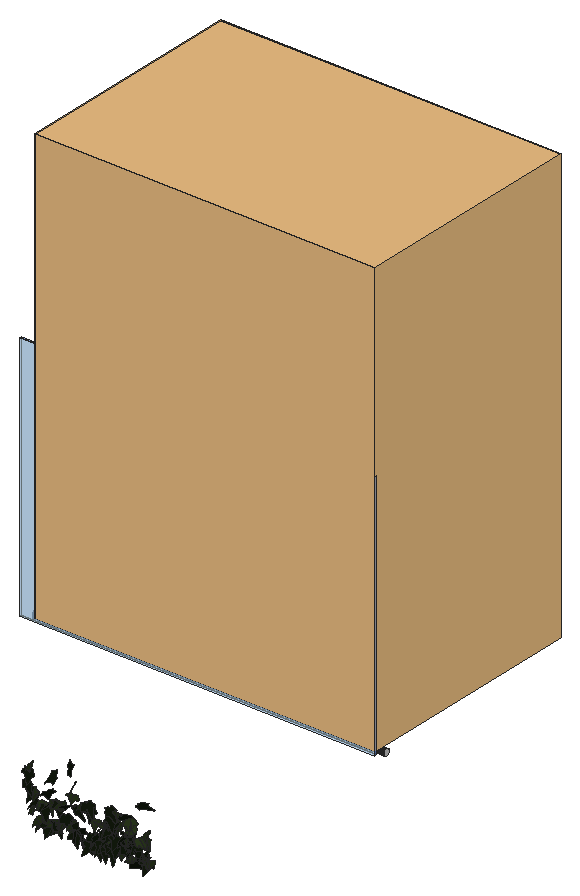
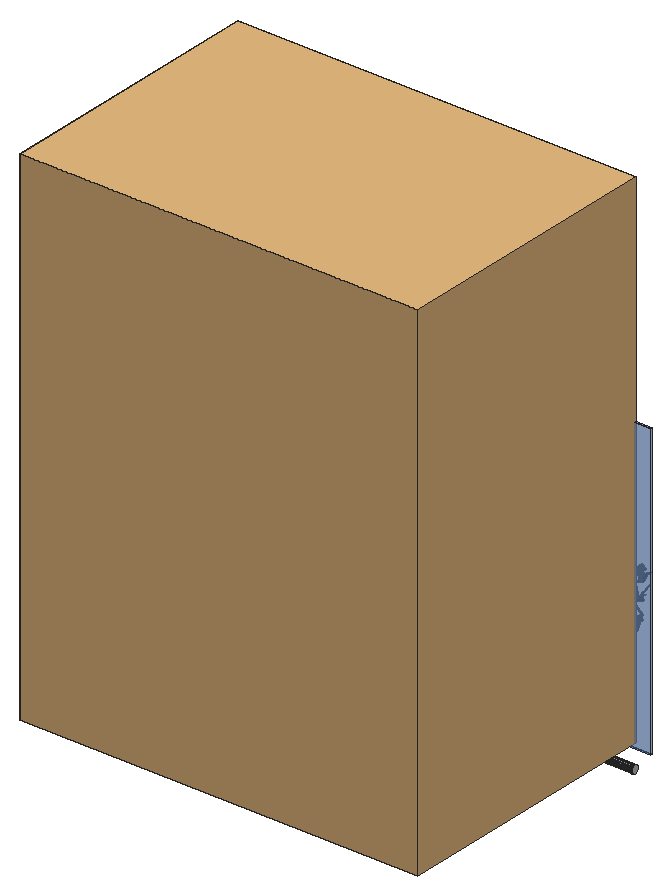
# SketchUp Ruby script. Lengths in inches.
U = 1.inch
M = Sketchup.active_model
def pt(a) = Geom::Point3d.new(a.map { |v| v * U })
def face(e, loops, mat)
  f = e.add_face(loops[0].map { |a| pt(a) })
  loops[1..].each { |l| e.add_face(l.map { |a| pt(a) }).erase! }
  f.material = f.back_material = mat if mat
  f
end
# faces: each face lists its corners as indices into pts; further lists are holes
def faces(e, pts, list, mat = nil) = list.each { |f| face(e, (f[0].is_a?(Array) ? f : [f]).map { |l| l.map { |i| pts[i] } }, mat) }
# xy, xz, yz: faces in a plane at the given z, y or x. An outline is a flat list of corners, or four numbers for a rectangle; further outlines are holes
def ring(l) = l.size == 4 ? [[l[0], l[1]], [l[2], l[1]], [l[2], l[3]], [l[0], l[3]]] : l.each_slice(2).to_a
def flat(e, list, mat, &to3) = list.each { |f| face(e, (f[0].is_a?(Array) ? f : [f]).map { |l| ring(l).map { |u, v| to3.(u, v) } }, mat) }
def xy(e, z, list, mat = nil) = flat(e, list, mat) { |x, y| [x, y, z] }
def xz(e, y, list, mat = nil) = flat(e, list, mat) { |x, z| [x, y, z] }
def yz(e, x, list, mat = nil) = flat(e, list, mat) { |y, z| [x, y, z] }
def lines(e, pts, list) = list.each { |a, b| e.add_line(pt(pts[a]), pt(pts[b])) }
# prism: a flat outline (further loops are holes) pulled along v
def prism(e, loops, v, mat = nil)
  f = face(e, loops, mat); d = Geom::Vector3d.new(v.map { |x| x * U })
  f.pushpull(f.normal.samedirection?(d) ? d.length : -d.length)
end
def box(e, o, s, mat = nil) = prism(e, [[o, [o[0] + s[0], o[1], o[2]], [o[0] + s[0], o[1] + s[1], o[2]], [o[0], o[1] + s[1], o[2]]]], [0, 0, s[2]], mat)
def at(x, y, z, deg = 0) = Geom::Transformation.translation(pt([x, y, z])) * Geom::Transformation.rotation(ORIGIN, Z_AXIS, deg.degrees)
def axes(o, x, y, z) = Geom::Transformation.new([*x, 0, *y, 0, *z, 0, *pt(o).to_a, 1])
def part(name) = M.definitions.add(name)
# library, detail: a bought-in or finely detailed component or shape, given as its bounding box
def library(name, o, s) = part(name).tap { |d| box(d.entities, o, s) }
def detail(e, o, s) = box(e.add_group.entities, o, s)
def put(e, d, t, mat = nil) = e.add_instance(d, t).tap { |i| i.material = mat if mat }
def group(e, t, mat = nil) = e.add_group.tap { |g| g.transformation = t; g.material = mat if mat }.entities
root = M.entities
M.materials.add("Glass Rail Metal").color = [192, 192, 192]
M.materials.add("[Translucent Glass Blue]").color = [100, 149, 237]
M.materials["[Translucent Glass Blue]"].alpha = 0.5
M.materials.add("[Translucent Glass Safety]").color = [204, 235, 244]
M.materials["[Translucent Glass Safety]"].alpha = 0.5
M.materials.add("efeu1").color = [18, 25, 13]
M.materials.add("efeu2").color = [43, 57, 29]
c1 = part("ivyleaf_9")
p = [[1.54,2.16,1.25],[1.36,2.04,1.19],[-0.21,0.99,0.68],[-0.71,1.11,0.82],[-0.85,0.86,0.67],[-0.8,0.17,0.21],
  [-0.9,-0.01,0.1],[-0.67,-0.16,-0.02],[-0.08,-0.08,-0.05],[-0.03,-0.6,-0.4],[0.65,-0.88,-0.66],[0.83,-0.6,-0.49],
  [1.29,-0.42,-0.43],[1.8125,-0.07,-0.26],[1.21,0.44,0.15]]
faces(c1.entities,p,[[0,1,2,3,4,5,6,7,8,9,10,11,12,13,14]],"efeu1")
c2 = part("ivyleaf_10")
p = [[0,0.5,-0.03],[-0.0625,2.02,-0.43],[-0.19,2.01,-0.46],[-0.54,1.05,-0.29],[-0.52,0.625,-0.18],[-0.83,0.76,-0.28],
  [-1.16,0.64,-0.33],[-1.15,0.33,-0.24],[-0.77,-0.39,0.02],[-0.3,-0.51,0.16],[0.04,-0.48,0.23],[-0.02,2.01,-0.4375],
  [-0.06,2.01,-0.43],[0.04,-0.49,0.23],[0.67,-0.49,0.14],[1.38,0.36,-0.2],[1.375,0.51,-0.24],[0.81,0.65,-0.19],
  [0.62,0.59,-0.15],[0.6,1.09,-0.28],[0.5,1.23,-0.31]]
faces(c2.entities,p,[[0,1,2,3,4,5,6,7,8,9,10],[11,12,0,13,14,15,16,17,18,19,20]],"efeu2")
c3 = library("Palm+in+pot",[-44.1,-44.03,0.04],[106.77,95.72,88.04])
prism(root,[[[506.55,181.67,254.4375],[506.55,181.84,254.35],[506.55,181.98,254.2],[506.55,182.09,254.02],[506.55,182.16,253.8125],[506.55,182.17,253.59],[506.55,182.14,253.375],[506.55,182.0625,253.18],[506.55,181.94,253.01],[506.55,181.79,252.88],[506.55,181.61,252.8],[506.55,181.43,252.78],[506.55,181.25,252.82],[506.55,181.08,252.91],[506.55,180.93,253.06],[506.55,180.83,253.24],[506.55,180.76,253.45],[506.55,180.75,253.67],[506.55,180.78,253.88],[506.55,180.86,254.09],[506.55,180.98,254.26],[506.55,181.13,254.38],[506.55,181.3,254.46],[506.55,181.49,254.48]]],[89.11,0,0],"Glass Rail Metal")
xy(root,254.7,[[506.22,177.2,595.99,177.79]],"[Translucent Glass Blue]")
xy(root,318.08,[[506.22,177.2,595.99,177.79]],"[Translucent Glass Blue]")
xz(root,177.2,[[506.22,254.7,595.99,318.08]],"[Translucent Glass Safety]")
xz(root,177.79,[[506.22,254.7,595.99,318.08]],"[Translucent Glass Blue]")
yz(root,506.22,[[177.2,254.7,177.79,318.08]],"[Translucent Glass Blue]")
yz(root,595.99,[[177.2,254.7,177.79,318.08]],"[Translucent Glass Blue]")
put(root,c1,axes([550.24,130.16,247.6875],[0.09934,-1.04431,-0.03336],[-0.02326,0.03129,-1.04883],[1.04459,0.10002,-0.02018]))
put(root,c1,axes([552.99,129.83,255.84],[-0.98011,0.38799,0.10195],[-0.09768,0.03022,-1.05409],[-0.38909,-0.98494,0.00782]))
put(root,c2,axes([571.6,130.2,247.97],[0.10661,-0.93081,0.4596],[0.10935,-0.44938,-0.93547],[1.03232,0.14373,0.05162]))
put(root,c2,axes([568.95,129.58,252.98],[-1.03024,0.12903,0.14532],[-0.14137,0.04033,-1.03805],[-0.13335,-1.03965,-0.02224]))
put(root,c1,axes([567.14,130.2,249.14],[-1.00045,-0.31834,0.02077],[-0.01948,-0.00727,-1.04987],[0.31842,-1.00064,0.00102]))
put(root,c1,axes([566.3,130.3,247.05],[-0.94363,-0.22886,-0.35753],[0.40475,-0.22235,-0.92594],[0.12797,-0.98429,0.2923]))
put(root,c1,axes([564.81,130.36,244.37],[-0.8856,-0.51614,-0.03288],[0.13113,-0.16102,-1.00431],[0.50028,-0.87146,0.20504]))
put(root,c2,axes([557.65,129.82,253.03],[-0.9508,-0.35541,0.30029],[-0.26159,-0.15666,-1.01368],[0.38479,-0.98471,0.05289]))
put(root,c2,axes([555.12,129.88,246.03],[0.2577,-1.02396,-0.05486],[-0.00277,0.05587,-1.05584],[1.02543,0.25749,0.01093]))
put(root,c2,axes([570.09,129.83,251.39],[0.15346,-1.03516,-0.1201],[-0.03109,0.11679,-1.04638],[1.04164,0.15599,-0.01354]))
put(root,c2,axes([548.8,129.43,244.65],[-0.29578,-0.77346,-0.63277],[0.29896,0.56119,-0.82572],[0.95355,-0.41587,0.06261]))
put(root,c1,axes([561.11,129.98,252.27],[0.06997,-0.99633,-0.43816],[0.1214,0.44347,-0.98902],[1.08163,0.01468,0.13935]))
put(root,c1,axes([566.86,130.26,251.14],[0.0567,-1.02927,-0.01108],[0.02641,0.01255,-1.03047],[1.02899,0.05639,0.02705]))
put(root,c1,axes([569.26,130.05,251.66],[-0.88669,0.40318,-0.38442],[0.32838,-0.20543,-0.97289],[-0.45,-0.94435,0.04751]))
put(root,c2,axes([569.13,129.95,250.08],[0.50057,-0.93252,-0.02492],[0.03234,0.04561,-1.05719],[0.93229,0.49911,0.05005]))
put(root,c1,axes([545.99,130.43,254.45],[-0.09848,-1.02006,0.18085],[-0.02567,-0.17921,-1.02477],[1.03565,-0.10144,-0.0082]))
put(root,c1,axes([568.11,130.33,245.47],[-0.19213,-1.02505,-0.02846],[-0.00573,0.03003,-1.04284],[1.02543,-0.19189,-0.01117]))
put(root,c1,axes([557.15,129.06,259.48],[0.1044,0.34296,-1.03239],[-0.9038,0.60458,0.10944],[0.60547,0.84333,0.34139]))
put(root,c1,axes([571.29,129.55,246.63],[0.29839,-0.08644,1.07907],[1.08247,0.01167,-0.29839],[0.01175,1.11951,0.08643]))
put(root,c1,axes([570.63,129.35,253.07],[0.79554,0.6998,-0.06753],[-0.03683,-0.06035,-1.05932],[-0.70209,0.79612,-0.02094]))
put(root,c1,axes([561.56,130.56,243.1875],[-0.70211,-0.7243,0.2139],[-0.05539,-0.24189,-1.00087],[0.7532,-0.69296,0.12579]))
put(root,c2,axes([571.95,129.85,252.26],[0.83512,0.66517,-0.01359],[-0.06187,0.05593,-1.06448],[-0.66242,0.83336,0.08228]))
put(root,c1,axes([563.97,130.14,243.72],[-0.30671,-0.89186,-0.40394],[0.14247,0.37813,-0.94307],[0.96865,-0.33801,0.0108]))
put(root,c1,axes([545.68,130.13,251.9375],[0.37961,-0.97219,-0.12719],[-0.028,0.12558,-1.04349],[0.98007,0.38015,0.01945]))
put(root,c2,axes([551.5625,130.22,248.26],[-0.56597,0.43778,-0.75759],[0.45618,-0.62229,-0.7004],[-0.74665,-0.71205,0.14633]))
put(root,c1,axes([568.4,130.51,246.99],[-0.65794,-0.79879,0.01773],[0.06576,-0.07703,-1.03005],[0.79627,-0.65366,0.09972]))
put(root,c1,axes([548.24,130.03,248.86],[-0.89328,0.47822,-0.14667],[0.1075,-0.10964,-1.01222],[-0.48852,-0.89858,0.04545]))
put(root,c1,axes([566.43,130.52,245.88],[-0.38609,-0.95523,0.09098],[-0.00099,-0.09768,-1.02969],[0.95955,-0.38445,0.03555]))
put(root,c1,axes([566.67,129.27,249.59],[-0.14747,0.85178,0.56979],[-0.19449,0.54193,-0.86048],[-1.00616,-0.2296,0.08282]))
put(root,c1,axes([555.58,130.11,247.46],[0.04784,-0.93068,-0.40341],[0.02332,0.40476,-0.93103],[1.01408,0.0346,0.04044]))
put(root,c1,axes([561.63,130.41,251.24],[-0.22718,-1.00478,-0.11456],[0.00067,0.11726,-1.02984],[1.01129,-0.2258,-0.02505]))
put(root,c2,axes([548.16,129.26,250.43],[0.08731,-0.3789,-0.99376],[0.00491,0.99724,-0.37979],[1.06354,0.0265,0.08333]))
put(root,c1,axes([565.15,130.1,247.03],[0.43038,-0.89576,-0.24795],[-0.05593,0.24779,-0.99226],[0.92776,0.43047,0.05521]))
put(root,c2,axes([576.23,129.625,244.88],[0.56664,-0.10726,-0.85706],[-0.65733,0.6114,-0.51111],[0.56033,0.82572,0.26711]))
put(root,c2,axes([565.6,129.78,244.29],[0.72786,-0.56503,-0.47277],[-0.2147,0.47305,-0.89592],[0.70475,0.72767,0.21533]))
put(root,c2,axes([572.62,130.12,243.38],[-0.32749,-0.02674,0.99814],[-0.95098,-0.31185,-0.32037],[0.30437,-1.00314,0.07299]))
put(root,c1,axes([566.69,130.13,253.07],[0.31485,-0.95105,-0.3112],[0.03288,0.3359,-0.99326],[1.00013,0.28835,0.13063]))
put(root,c1,axes([546.93,130.73,250.14],[-0.42065,-0.86898,0.32729],[-0.07642,-0.32569,-0.96296],[0.92542,-0.42189,0.06925]))
put(root,c2,axes([557.26,129.83,246.52],[-0.09862,-0.99063,-0.37102],[0.12773,0.35875,-0.99183],[1.05009,-0.13668,0.08579]))
put(root,c2,axes([572.19,130.26,249.91],[0.50779,0.551,0.72978],[-0.50399,-0.52789,0.74925],[0.76301,-0.71538,0.00922]))
put(root,c1,axes([550.91,130.58,243.86],[-0.43171,-0.93763,-0.01567],[0.0485,-0.0051,-1.03121],[0.9365,-0.43197,0.04618]))
put(root,c2,axes([560.18,129.84,251.85],[-0.4836,-0.88252,-0.33517],[0.13583,0.30762,-1.00597],[0.9342,-0.50157,-0.02724]))
put(root,c2,axes([554.5,130.04,249.96],[-0.30229,-1.00367,-0.10117],[0.0285,0.09708,-1.04821],[1.00836,-0.30363,-0.00071]))
put(root,c1,axes([572.55,129.93,248.24],[-0.72246,0.73124,0.0075],[-0.00606,0.00456,-1.02794],[-0.73125,-0.72248,0.0011]))
put(root,c2,axes([574.5,129.75,248.84],[0.67457,0.59612,0.56255],[0.36186,0.43713,-0.89713],[-0.73545,0.76185,0.07457]))
put(root,c1,axes([551.11,129.6875,251.72],[0.3859,0.93418,-0.24925],[-0.10291,-0.22716,-1.01071],[-0.96136,0.3993,0.00814]))
put(root,c1,axes([553.16,130.21,244.79],[0.43009,-0.90853,-0.30046],[-0.13504,0.26849,-1.00517],[0.94735,0.45074,-0.00687]))
put(root,c1,axes([565.18,130.51,243.32],[-0.09038,-0.99865,-0.13127],[0.0749,0.12477,-1.00076],[1.00445,-0.09916,0.06281]))
put(root,c1,axes([573.55,130.59,247.3125],[-0.90884,-0.46811,-0.04788],[0.04546,0.01629,-1.02229],[0.46835,-0.90996,0.00632]))
put(root,c1,axes([573.58,130.05,245.82],[0.73663,-0.69796,-0.23578],[-0.06524,0.27031,-1.00401],[0.73382,0.72467,0.14742]))
put(root,c1,axes([564.57,129.51,247.99],[-0.07502,0.97908,0.3179],[-0.14942,0.30501,-0.97464],[-1.01849,-0.11686,0.11957]))
put(root,c2,axes([549.67,130.31,248.26],[0.71288,0.31821,-0.67189],[-0.66784,-0.13488,-0.77246],[-0.32663,0.97028,0.11297]))
put(root,c1,axes([557.6,130.42,244.22],[-0.01445,-0.98694,-0.28146],[0.08974,0.27919,-0.9836],[1.02236,-0.03845,0.08236]))
put(root,c2,axes([572.05,129.8,251.24],[0.39448,-0.78842,-0.58895],[-0.05803,0.61477,-0.86184],[0.98239,0.3529,0.18558]))
put(root,c1,axes([565.52,130.83,248.27],[-0.12512,-0.40963,0.92801],[0.34423,-0.89671,-0.3494],[0.9542,0.26977,0.24773]))
put(root,c1,axes([553.6,130.53,249.55],[-0.16886,-0.98327,-0.21084],[0.05873,0.20378,-0.9974],[1.00391,-0.17732,0.02289]))
put(root,c1,axes([561.5,130.07,250.78],[0.705,-0.71626,-0.42276],[-0.28815,0.30954,-1.00496],[0.78021,0.76153,0.01086]))
put(root,c1,axes([576.14,130.05,246.39],[-0.73215,0.73903,0.00971],[-0.00851,0.00523,-1.04029],[-0.73904,-0.7322,0.00237]))
put(root,c2,axes([553.25,130.34,245.14],[0.72581,-0.56514,0.47445],[0.57285,0.01206,-0.86196],[0.46511,0.86704,0.32124]))
put(root,c1,axes([573.36,129.52,243.26],[0.62148,0.92076,0.13104],[0.07303,0.10881,-1.11087],[-0.92716,0.62576,0.00034]))
put(root,c1,axes([558.13,129.57,244.32],[0.13552,0.03149,-1.0264],[-0.8725,0.54947,-0.09834],[0.5415,0.87746,0.09842]))
put(root,c2,axes([564.92,130.07,247.33],[0.4751,-0.85711,-0.33513],[-0.0044,0.37503,-0.9654],[0.92029,0.44427,0.16839]))
put(root,c2,axes([552.51,130.125,249.82],[-0.93419,-0.01619,-0.47853],[0.47841,0.01137,-0.93433],[0.01959,-1.04956,-0.00274]))
put(root,c2,axes([549.15,130.1875,247.85],[-0.97172,-0.29226,0.14895],[-0.1504,-0.01691,-1.01436],[0.29152,-0.98292,-0.02683]))
put(root,c2,axes([575.86,130.41,250.68],[-0.00324,-1.03693,0.03783],[-0.01405,-0.03778,-1.03684],[1.03752,-0.00375,-0.01392]))
put(root,c1,axes([566.8125,130.77,243.17],[0.11776,-1.0127,0.1095],[0.00095,-0.11012,-1.01945],[1.0186,0.11718,-0.01171]))
put(root,c1,axes([557.48,129.43,254.48],[-0.01253,0.65977,0.8441],[0.02028,0.84416,-0.65951],[-1.07116,0.00827,-0.02236]))
put(root,c1,axes([571.49,130.27,248.78],[0.72539,-0.74514,-0.11981],[0.09076,0.2511,-1.01217],[0.74923,0.69101,0.23861]))
put(root,c2,axes([562.95,130.62,248.72],[-0.54099,-0.81162,0.33309],[-0.01016,-0.38551,-0.95584],[0.87725,-0.50498,0.19434]))
put(root,c1,axes([574.63,129.67,256.87],[0.99918,0.40498,0.44983],[0.40536,0.19702,-1.07777],[-0.44949,1.07792,0.02798]))
put(root,c1,axes([552.08,130.4,244.81],[0.77952,-0.63543,0.21329],[0.22294,-0.06272,-1.00164],[0.63211,0.80574,0.09024]))
put(root,c1,axes([561.97,130.47,245.39],[0.07395,-0.93447,-0.38706],[0.08161,0.39234,-0.93162],[1.00816,0.03678,0.1038]))
put(root,c2,axes([546.41,130.3,256.1],[0.04439,-1.03146,-0.17572],[-0.03298,0.17441,-1.03211],[1.0458,0.04928,-0.02509]))
put(root,c2,axes([576.04,130.46,244.95],[0.46544,-0.92877,-0.04513],[-0.00403,0.04845,-1.03871],[0.92985,0.4651,0.01808]))
put(root,c2,axes([576.38,130.04,248.875],[-0.38627,0.93003,0.29023],[-0.25128,0.20654,-0.99629],[-0.9413,-0.43678,0.14686]))
put(root,c1,axes([563.375,130.67,245.52],[-0.1422,0.58015,-0.82585],[0.09855,-0.82204,-0.59445],[-1.00444,-0.16279,0.05859]))
put(root,c2,axes([554.03,130.08,244.5],[0.4468,-0.8008,-0.51243],[-0.0153,0.56007,-0.88859],[0.9506,0.38541,0.22655]))
put(root,c1,axes([569.43,130.45,248.46],[0.7165,-0.46528,0.58847],[0.57612,-0.17992,-0.84372],[0.48049,0.90956,0.13413]))
put(root,c2,axes([553.21,130.45,244.72],[-0.16551,-0.98816,-0.04855],[0.01138,0.04732,-1.00192],[0.98929,-0.16586,0.0034]))
put(root,c1,axes([560.07,130.55,243.03],[0.57214,-0.80984,0.02263],[0.17429,0.09599,-0.97165],[0.79119,0.56448,0.19769]))
put(root,c1,axes([570.04,130.52,245.34],[0.42285,-0.89334,-0.27629],[-0.03644,0.28725,-0.98456],[0.93438,0.41548,0.08663]))
put(root,c2,axes([576.54,130.6,244.15],[-0.4656,-0.87306,0.18737],[-0.07952,-0.16994,-0.98941],[0.8894,-0.47225,0.00963]))
put(root,c1,axes([561.82,130.85,244.6],[0.15714,-1.01272,0.00254],[0.00023,-0.00253,-1.02483],[1.01272,0.15714,-0.00016]))
put(root,c1,axes([575.77,130.98,243.84],[-0.65474,-0.77245,-0.08162],[0.12008,0.00481,-1.00875],[0.76741,-0.65979,0.0882]))
put(root,c1,axes([550.98,129.98,248.65],[-0.13713,1.01208,0.06521],[-0.06236,0.05726,-1.0199],[-1.01226,-0.14063,0.054]))
put(root,c2,axes([557.03,130.27,244.4],[-0.127,-0.95611,-0.36612],[0.1127,0.35363,-0.96258],[1.01759,-0.15849,0.06092]))
put(root,c1,axes([557.2,130.54,246.49],[0.66035,-0.80385,-0.22151],[-0.13104,0.179,-1.04024],[0.82345,0.67312,0.0121]))
put(root,c2,axes([548.28,130.19,243.23],[0.35646,-0.77203,-0.55109],[-0.07338,0.56451,-0.83829],[0.9457,0.3348,0.14268]))
put(root,c2,axes([565.59,130.8125,248.38],[-0.17166,-0.00508,-1.008],[-0.97549,-0.25681,0.16741],[-0.254,0.98973,0.03827]))
put(root,c1,axes([557.83,130.53,249.82],[0.67655,-0.76888,-0.15854],[0.0511,0.25198,-1.00395],[0.78339,0.64758,0.20241]))
put(root,c1,axes([567.3,130.1875,248.89],[0.67735,-0.36285,-0.81506],[-0.73628,0.3506,-0.76795],[0.50386,1.0001,-0.02649]))
put(root,c1,axes([565.95,130.75,247.82],[0.10709,-0.17692,1.00541],[0.83153,-0.57133,-0.18911],[0.5922,0.83421,0.08371]))
put(root,c2,axes([546.85,130.53,246.27],[0.1122,-0.99591,-0.24169],[0.02968,0.24619,-1.00067],[1.02438,0.10195,0.05546]))
put(root,c2,axes([565.3,130.69,245.28],[0.1124,-1.02114,-0.04419],[-0.02913,0.04123,-1.02701],[1.02168,0.11352,-0.02442]))
put(root,c2,axes([572.04,130.54,247.77],[0.06373,-0.98569,-0.28303],[0.03234,0.28537,-0.98654],[1.02501,0.05228,0.04873]))
put(root,c2,axes([570.94,130.64,245.06],[0.8748,-0.54541,0.04342],[0.17788,0.20609,-0.99525],[0.51741,0.85129,0.26876]))
put(root,c1,axes([553.01,131.14,243.77],[-0.94144,-0.31371,0.20184],[-0.17823,-0.10309,-0.9915],[0.3277,-0.9573,0.04062]))
put(root,c2,axes([568.84,130.49,243.88],[-0.96023,0.28164,0.17703],[-0.16123,0.07902,-1.00023],[-0.29098,-0.97321,-0.02998]))
put(root,c2,axes([551.28,130.73,244.55],[-0.72499,-0.71478,0.07784],[-0.05228,-0.05784,-1.01809],[0.7171,-0.72686,0.00447]))
put(root,c1,axes([572.16,130.14,246.18],[-0.15318,0.9663,0.3158],[-0.22715,0.27876,-0.96313],[-0.99089,-0.21328,0.17197]))
put(root,c2,axes([551.84,130.92,243.89],[0.60508,-0.80814,0.14738],[0.12723,-0.08864,-1.00841],[0.81155,0.61643,0.04821]))
put(root,c2,axes([567.0625,130.56,246],[0.75491,0.68437,0.19408],[0.07366,0.20627,-1.01388],[-0.70754,0.75167,0.10152]))
put(root,c2,axes([565.04,130.5,245.34],[0.97215,-0.03657,-0.36736],[-0.31815,0.44192,-0.88592],[0.18728,0.9406,0.40195]))
put(root,c2,axes([551.34,131.02,243.55],[-0.36505,-0.92195,0.21443],[0.0047,-0.23158,-0.98771],[0.94654,-0.35441,0.0876]))
put(root,c1,axes([574.42,130.23,244.55],[0.78714,0.65891,0.10361],[0.08923,0.0548,-1.02642],[-0.66101,0.79204,-0.01518]))
put(root,c2,axes([560.95,130.7,243.62],[0.8726,-0.52387,-0.15282],[0.06629,0.38784,-0.951],[0.54166,0.79647,0.36257]))
put(root,c2,axes([550.81,130.95,242.86],[-0.15781,-1.0057,0.01739],[-0.01837,-0.01472,-1.01789],[1.00569,-0.15808,-0.01587]))
put(root,c2,axes([554.41,130.54,245.28],[0.07841,-0.87053,-0.59265],[-0.05489,0.59011,-0.87405],[1.05168,0.0957,-0.00143]))
put(root,c1,axes([565.84,130.7,247.38],[0.89522,-0.4395,-0.21401],[-0.1196,0.23604,-0.98507],[0.47398,0.88967,0.15563]))
put(root,c1,axes([559.61,130.25,243.2],[0.24724,0.24996,-0.93266],[-0.8711,0.47307,-0.10414],[0.41655,0.84094,0.33581]))
put(root,c2,axes([562.23,131.01,243.26],[0.97937,-0.22116,-0.12808],[-0.11023,0.0921,-1.00192],[0.23057,0.9834,0.06503]))
put(root,c1,axes([565.25,130.74,248.31],[0.80415,-0.53048,-0.3463],[-0.19176,0.32952,-0.95007],[0.60379,0.81117,0.15947]))
put(root,c1,axes([564.38,130.83,243.18],[-0.7,0.74436,0.00306],[-0.01367,-0.00866,-1.02167],[-0.74424,-0.69995,0.0159]))
put(root,c1,axes([554.18,130.36,248.75],[0.62533,0.01251,0.83477],[0.70517,0.55041,-0.53649],[-0.44693,0.88596,0.32151]))
put(root,c2,axes([557.59,130.96,244.14],[0.17477,-0.02371,-1.04456],[-1.01096,0.26363,-0.17513],[0.26387,1.02575,0.02087]))
put(root,c2,axes([575.7,131.08,243.625],[0.64659,-0.77001,-0.12744],[0.0518,0.20746,-0.99071],[0.77876,0.62552,0.17171]))
put(root,c1,axes([558.2,130.79,245.05],[0.59269,0.74385,-0.47283],[-0.28383,-0.37837,-0.95103],[-0.83446,0.65703,-0.01236]))
put(root,c2,axes([548.94,131.38,244.38],[-0.82923,-0.45287,0.31982],[-0.09857,-0.44583,-0.88686],[0.54558,-0.76886,0.32588]))
put(root,c2,axes([574.53,130.89,244.48],[-0.72225,0.69827,0.15516],[-0.17429,0.04206,-1.00058],[-0.69374,-0.73753,0.08984]))
put(root,c1,axes([571.49,130.29,244.72],[0.09977,0.79581,0.6446],[0.09462,0.63772,-0.80196],[-1.01974,0.13703,-0.01135]))
put(root,c1,axes([569.09,130.27,246.03],[0.2935,0.36321,1.03584],[0.53939,0.88612,-0.46354],[-0.95601,0.61146,0.05647]))
put(root,c1,axes([571.7,130.64,244.16],[0.07727,0.24441,-0.99432],[-0.97757,0.31424,0.00128],[0.30459,0.94652,0.25633]))
put(root,c1,axes([561.68,131.4,242.91],[0.14276,-0.10002,0.98469],[0.70138,0.71219,-0.02934],[-0.69835,0.69483,0.17182]))
put(root,c3,axes([545.45,204.27,255.63],[0.80651,0,0],[0,0.615,0],[0,0,1.24722]))
